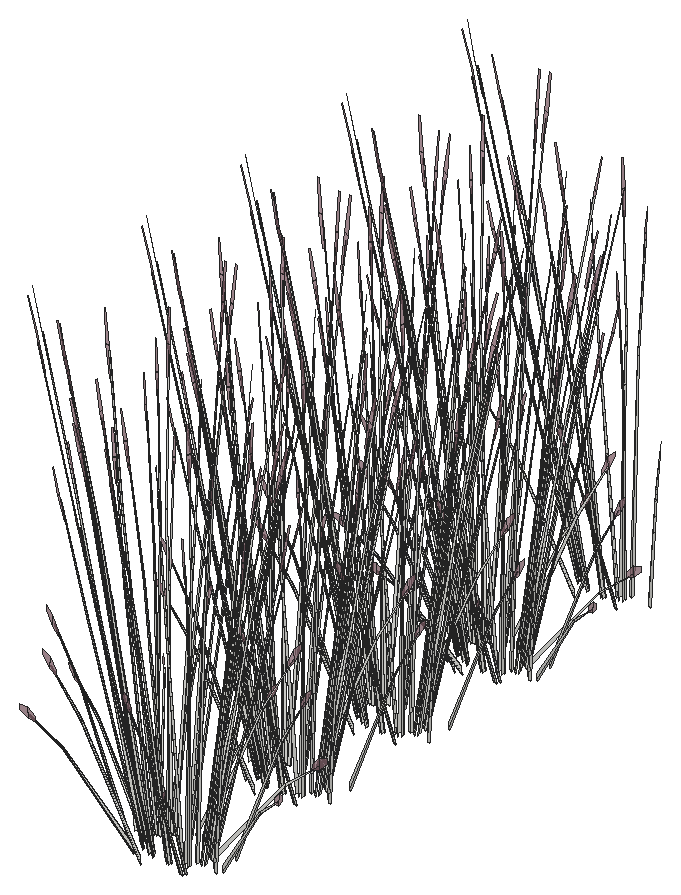
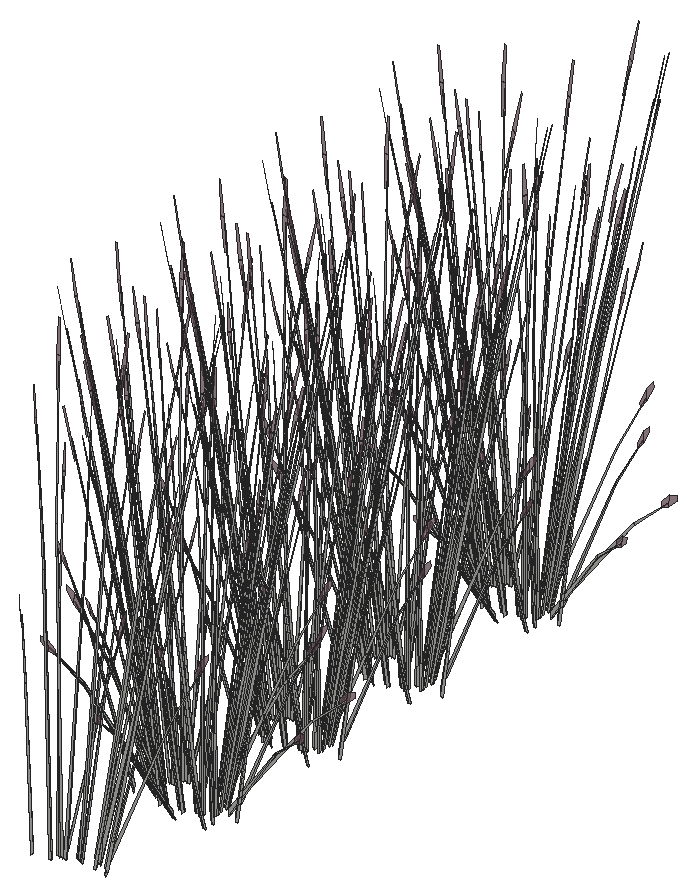
# SketchUp Ruby script. Lengths in inches.
U = 1.inch
M = Sketchup.active_model
def pt(a) = Geom::Point3d.new(a.map { |v| v * U })
def face(e, loops, mat)
  f = e.add_face(loops[0].map { |a| pt(a) })
  loops[1..].each { |l| e.add_face(l.map { |a| pt(a) }).erase! }
  f.material = f.back_material = mat if mat
  f
end
# faces: each face lists its corners as indices into pts; further lists are holes
def faces(e, pts, list, mat = nil) = list.each { |f| face(e, (f[0].is_a?(Array) ? f : [f]).map { |l| l.map { |i| pts[i] } }, mat) }
# xy, xz, yz: faces in a plane at the given z, y or x. An outline is a flat list of corners, or four numbers for a rectangle; further outlines are holes
def ring(l) = l.size == 4 ? [[l[0], l[1]], [l[2], l[1]], [l[2], l[3]], [l[0], l[3]]] : l.each_slice(2).to_a
def flat(e, list, mat, &to3) = list.each { |f| face(e, (f[0].is_a?(Array) ? f : [f]).map { |l| ring(l).map { |u, v| to3.(u, v) } }, mat) }
def xy(e, z, list, mat = nil) = flat(e, list, mat) { |x, y| [x, y, z] }
def xz(e, y, list, mat = nil) = flat(e, list, mat) { |x, z| [x, y, z] }
def yz(e, x, list, mat = nil) = flat(e, list, mat) { |y, z| [x, y, z] }
def lines(e, pts, list) = list.each { |a, b| e.add_line(pt(pts[a]), pt(pts[b])) }
# prism: a flat outline (further loops are holes) pulled along v
def prism(e, loops, v, mat = nil)
  f = face(e, loops, mat); d = Geom::Vector3d.new(v.map { |x| x * U })
  f.pushpull(f.normal.samedirection?(d) ? d.length : -d.length)
end
def box(e, o, s, mat = nil) = prism(e, [[o, [o[0] + s[0], o[1], o[2]], [o[0] + s[0], o[1] + s[1], o[2]], [o[0], o[1] + s[1], o[2]]]], [0, 0, s[2]], mat)
def at(x, y, z, deg = 0) = Geom::Transformation.translation(pt([x, y, z])) * Geom::Transformation.rotation(ORIGIN, Z_AXIS, deg.degrees)
def axes(o, x, y, z) = Geom::Transformation.new([*x, 0, *y, 0, *z, 0, *pt(o).to_a, 1])
def part(name) = M.definitions.add(name)
# library, detail: a bought-in or finely detailed component or shape, given as its bounding box
def library(name, o, s) = part(name).tap { |d| box(d.entities, o, s) }
def detail(e, o, s) = box(e.add_group.entities, o, s)
def put(e, d, t, mat = nil) = e.add_instance(d, t).tap { |i| i.material = mat if mat }
def group(e, t, mat = nil) = e.add_group.tap { |g| g.transformation = t; g.material = mat if mat }.entities
root = M.entities
M.materials.add("LightPink_Translucent").color = [144, 107, 117]
M.materials["LightPink_Translucent"].alpha = 0.75
c1 = part("blade")
p = [[2.15,0.21,22],[0,0.17,0],[0.09,0.45,0],[2.18,0.31,22],[2.29,0.31,22],[0.38,0.45,0],
  [2.48,0.24,33],[2.49,0.24,33],[2.48,0.22,33]]
faces(c1.entities,p,[[0,1,2,3],[4,5,2,3],[6,3,4,7],[8,0,3,6]])
c2 = part("seeds")
p = [[0.3,-0.1,1.38],[-0.01,-0.03,1.59],[-0.01,-0.03,0.03],[0.14,-0.07,-0.07],[0.29,-0.03,3],[0.15,0.01,3.11]]
faces(c2.entities,p,[[0,1,2,3],[1,0,4,5]],"LightPink_Translucent")
c3 = part("blade with seeds")
put(c3.entities,c1,at(0,0,0))
put(c3.entities,c2,axes([2.4,0.25,30.99],[1.5799,-0.05474,1.17369],[-0.12525,1.92788,0.29478],[-0.07173,-0.02425,1.56792]))
put(root,c3,axes([335.89,344.47,52.17],[-0.00487,-0.07777,1.54581],[-0.41166,-0.22476,-0.24447],[0.06364,-0.13625,0.12397]))
put(root,c3,axes([335.78,344.1875,52.16],[-0.05128,0.02985,1.56736],[-0.5024,-0.1007,-0.1481],[-0.01819,-0.13025,0.27737]))
put(root,c3,axes([333.05,343.62,52.16],[-0.00942,0.04684,1.56736],[-0.46458,0.16998,-0.1481],[-0.13671,-0.08689,0.27737]))
put(root,c3,axes([332.94,344.45,52.5],[0.56246,-0.10044,0.47505],[0.09762,0.39398,0.3917],[-0.13228,-0.11611,0.983]))
put(root,c3,axes([334.22,344.52,52.18],[0.49753,0.10215,0.42415],[-0.17013,0.33585,0.34973],[-0.0299,-0.13207,0.87768]))
put(root,c3,axes([334.35,344.49,52.18],[0.37205,-0.1328,0.05682],[0.18211,0.24217,0.44729],[-0.03593,-0.10675,0.68204]))
put(root,c3,axes([333.07,344.53,52.18],[0.22948,-0.24822,0.05682],[0.32679,0.14452,0.44729],[-0.10565,-0.07958,0.68204]))
put(root,c3,axes([334.21,344.77,52.46],[-0.15222,0.30049,0.31292],[-0.44409,-0.08764,-0.40398],[-0.04072,-0.12098,0.77298]))
put(root,c3,axes([335.34,344.89,52.18],[0.35954,0.26661,0.42415],[-0.38183,0.22994,0.34973],[0.06632,-0.12508,0.87768]))
put(root,c3,axes([333.18,344.51,52.8],[-0.33698,0.3746,-0.12034],[-0.48801,-0.21581,-0.66795],[-0.16964,-0.10584,1.01494]))
put(root,c3,axes([335.48,344.92,52.18],[0.41493,0.01821,0.05682],[-0.01138,0.27493,0.44729],[0.04342,-0.10531,0.68204]))
put(root,c3,axes([335.17,345.11,52.46],[-0.34164,0.20573,0.31292],[-0.3234,-0.23491,-0.40398],[0.04921,-0.11936,0.77298]))
put(root,c3,axes([331.88,344.4,52.17],[-0.10864,-0.00276,1.54581],[-0.34587,0.27582,-0.24447],[-0.18454,-0.05636,0.12397]))
put(root,c3,axes([333.14,344.82,52.46],[0.07798,0.31474,0.31292],[-0.44579,0.08311,-0.40398],[-0.11974,-0.09019,0.77298]))
put(root,c3,axes([331.8,345.02,52.5],[0.41698,-0.28837,0.47505],[0.35962,0.30624,0.3917],[-0.19563,-0.05319,0.983]))
put(root,c3,axes([337.14,345.68,52.16],[-0.06595,-0.00297,1.56736],[-0.27386,-0.31799,-0.1481],[0.10998,-0.10455,0.27737]))
put(root,c3,axes([331.99,345.02,52.18],[0.02542,-0.29714,0.05682],[0.38391,0.00815,0.44729],[-0.14706,-0.03109,0.68204]))
put(root,c3,axes([335.76,345.74,52.46],[-0.43951,0.05584,0.31292],[-0.11606,-0.31924,-0.40398],[0.12595,-0.08575,0.77298]))
put(root,c3,axes([336.16,345.69,52.18],[0.34663,0.16434,0.05682],[-0.20181,0.23402,0.44729],[0.11113,-0.07566,0.68204]))
put(root,c3,axes([336.0625,345.62,52.18],[0.12522,0.35963,0.42415],[-0.49122,0.06241,0.34973],[0.14477,-0.08458,0.87768]))
put(root,c3,axes([337.39,346.06,52.17],[0.07006,-0.05952,1.54581],[-0.08968,-0.3651,-0.24447],[0.1758,-0.06922,0.12397]))
put(root,c3,axes([331.47,344.63,52.16],[0.03743,0.039,1.56736],[-0.18045,0.35054,-0.1481],[-0.18276,0.00254,0.27737]))
put(root,c3,axes([332.25,345.24,52.46],[0.28729,0.24465,0.31292],[-0.32804,0.23159,-0.40398],[-0.16667,-0.03524,0.77298]))
put(root,c3,axes([335.83,346.5,52.46],[-0.41962,-0.10901,0.31292],[0.12239,-0.31802,-0.40398],[0.16894,-0.02916,0.77298]))
put(root,c3,axes([331.4375,345.92,52.18],[0.14265,-0.35629,0.42415],[0.46898,0.12183,0.34973],[-0.18443,0.02141,0.87768]))
put(root,c3,axes([331.4,345.83,52.18],[-0.18545,-0.26643,0.05682],[0.33817,-0.13041,0.44729],[-0.14907,0.02573,0.68204]))
put(root,c3,axes([336.21,346.6,52.18],[0.18545,0.26643,0.05682],[-0.33817,0.13041,0.44729],[0.14907,-0.02573,0.68204]))
put(root,c3,axes([336.18,346.51,52.18],[-0.14265,0.35629,0.42415],[-0.46898,-0.12183,0.34973],[0.18443,-0.02141,0.87768]))
put(root,c3,axes([331.78,345.93,52.46],[0.41962,0.10901,0.31292],[-0.12239,0.31802,-0.40398],[-0.16894,0.02916,0.77298]))
put(root,c3,axes([337.02,347.66,52.16],[-0.04566,-0.03421,1.56736],[0.09987,-0.36669,-0.1481],[0.17984,-0.02343,0.27737]))
put(root,c3,axes([331.08,346.17,52.17],[-0.08245,0.05073,1.54581],[0.00701,0.37067,-0.24447],[-0.18899,0.0482,0.12397]))
put(root,c3,axes([335.36,347.19,52.46],[-0.28729,-0.24465,0.31292],[0.32804,-0.23159,-0.40398],[0.16667,0.03524,0.77298]))
put(root,c3,axes([335.88,347.11,52.17],[0.10831,-0.00661,1.54581],[0.29709,-0.30358,-0.24447],[0.19266,0.04007,0.12397]))
put(root,c3,axes([331.55,346.8125,52.18],[-0.12522,-0.35963,0.42415],[0.49122,-0.06241,0.34973],[-0.14477,0.08458,0.87768]))
put(root,c3,axes([331.45,346.74,52.18],[-0.34663,-0.16434,0.05682],[0.20181,-0.23402,0.44729],[-0.11113,0.07566,0.68204]))
put(root,c3,axes([331.85,346.69,52.46],[0.43951,-0.05584,0.31292],[0.11606,0.31924,-0.40398],[-0.12595,0.08575,0.77298]))
put(root,c3,axes([330.16,346.55,52.16],[0.06444,0.01048,1.56736],[0.19934,0.34525,-0.1481],[-0.13191,0.09062,0.27737]))
put(root,c3,axes([335.62,347.41,52.18],[-0.02542,0.29714,0.05682],[-0.38391,-0.00815,0.44729],[0.14706,0.03109,0.68204]))
put(root,c3,axes([335.65,347.32,52.18],[-0.3723,0.25748,0.42415],[-0.32109,-0.27343,0.34973],[0.17467,0.04749,0.87768]))
put(root,c3,axes([330.85,347.6,52.99],[0.44556,0.1043,-0.05733],[-0.13706,0.32103,-0.25992],[-0.07288,0.04874,0.85731]))
put(root,c3,axes([334.47,347.62,52.46],[-0.07798,-0.31474,0.31292],[0.44579,-0.08311,-0.40398],[0.11974,0.09019,0.77298]))
put(root,c3,axes([332.45,347.33,52.46],[0.34164,-0.20573,0.31292],[0.3234,0.23491,-0.40398],[-0.04921,0.11936,0.77298]))
put(root,c3,axes([334.04,348.06,52.16],[0.00149,-0.04731,1.56736],[0.4327,-0.20872,-0.1481],[0.1503,0.0745,0.27737]))
put(root,c3,axes([332.14,347.51,52.18],[-0.41493,-0.01821,0.05682],[0.01138,-0.27493,0.44729],[-0.04342,0.10531,0.68204]))
put(root,c3,axes([332.27,347.54,52.18],[-0.35954,-0.26661,0.42415],[0.38183,-0.22994,0.34973],[-0.06632,0.12508,0.87768]))
put(root,c3,axes([333.4,347.67,52.46],[0.15222,-0.30049,0.31292],[0.44409,0.08764,-0.40398],[0.04072,0.12098,0.77298]))
put(root,c3,axes([334.54,347.9,52.18],[-0.22948,0.24822,0.05682],[-0.32679,-0.14452,0.44729],[0.10565,0.07958,0.68204]))
put(root,c3,axes([334,348.74,52.99],[0.34892,-0.22417,-0.05733],[0.3197,0.24551,-0.25992],[0.02251,0.06957,0.85731]))
put(root,c3,axes([334.64,347.83,52.18],[-0.5022,0.08967,0.42415],[-0.08716,-0.35177,0.34973],[0.11811,0.10367,0.87768]))
put(root,c3,axes([333.27,347.9375,52.18],[-0.37205,0.1328,0.05682],[-0.18211,-0.24217,0.44729],[0.03593,0.10675,0.68204]))
put(root,c3,axes([331.09,347.56,52.17],[-0.01255,0.07733,1.54581],[0.35618,0.269,-0.24447],[-0.09325,0.12721,0.12397]))
put(root,c3,axes([332.23,347.38,52.77],[0.55492,0.01936,-0.11927],[-0.01517,0.36657,-0.66198],[-0.03855,0.14118,1.00587]))
put(root,c3,axes([333.4,347.91,52.47],[-0.49753,-0.10215,0.47081],[0.17013,-0.33585,0.3882],[0.0299,0.13207,0.97422]))
put(root,c3,axes([331.05,348.35,52.16],[0.05728,-0.02359,1.56736],[0.47345,0.15692,-0.1481],[-0.01113,0.13066,0.27737]))
put(root,c3,axes([333.14,348.51,52.17],[0.064,0.06292,1.54581],[0.51651,0.02472,-0.24447],[0.05194,0.13877,0.12397]))
put(root,c3,axes([335.78,354.91,52.16],[-0.05128,0.02985,1.56736],[-0.5024,-0.1007,-0.1481],[-0.01819,-0.13025,0.27737]))
put(root,c3,axes([333.05,354.34,52.16],[-0.00942,0.04684,1.56736],[-0.46458,0.16998,-0.1481],[-0.13671,-0.08689,0.27737]))
put(root,c3,axes([332.94,355.17,52.5],[0.56246,-0.10044,0.47505],[0.09762,0.39398,0.3917],[-0.13228,-0.11611,0.983]))
put(root,c3,axes([334.22,355.24,52.18],[0.49753,0.10215,0.42415],[-0.17013,0.33585,0.34973],[-0.0299,-0.13207,0.87768]))
put(root,c3,axes([334.35,355.22,52.18],[0.37205,-0.1328,0.05682],[0.18211,0.24217,0.44729],[-0.03593,-0.10675,0.68204]))
put(root,c3,axes([333.07,355.25,52.18],[0.22948,-0.24822,0.05682],[0.32679,0.14452,0.44729],[-0.10565,-0.07958,0.68204]))
put(root,c3,axes([334.21,355.49,52.46],[-0.15222,0.30049,0.31292],[-0.44409,-0.08764,-0.40398],[-0.04072,-0.12098,0.77298]))
put(root,c3,axes([335.34,355.62,52.18],[0.35954,0.26661,0.42415],[-0.38183,0.22994,0.34973],[0.06632,-0.12508,0.87768]))
put(root,c3,axes([333.18,355.23,52.8],[-0.33698,0.3746,-0.12034],[-0.48801,-0.21581,-0.66795],[-0.16964,-0.10584,1.01494]))
put(root,c3,axes([335.48,355.64,52.18],[0.41493,0.01821,0.05682],[-0.01138,0.27493,0.44729],[0.04342,-0.10531,0.68204]))
put(root,c3,axes([335.17,355.83,52.46],[-0.34164,0.20573,0.31292],[-0.3234,-0.23491,-0.40398],[0.04921,-0.11936,0.77298]))
put(root,c3,axes([333.14,355.54,52.46],[0.07798,0.31474,0.31292],[-0.44579,0.08311,-0.40398],[-0.11974,-0.09019,0.77298]))
put(root,c3,axes([331.8,355.74,52.5],[0.41698,-0.28837,0.47505],[0.35962,0.30624,0.3917],[-0.19563,-0.05319,0.983]))
put(root,c3,axes([337.14,356.4,52.16],[-0.06595,-0.00297,1.56736],[-0.27386,-0.31799,-0.1481],[0.10998,-0.10455,0.27737]))
put(root,c3,axes([331.99,355.74,52.18],[0.02542,-0.29714,0.05682],[0.38391,0.00815,0.44729],[-0.14706,-0.03109,0.68204]))
put(root,c3,axes([335.76,356.46,52.46],[-0.43951,0.05584,0.31292],[-0.11606,-0.31924,-0.40398],[0.12595,-0.08575,0.77298]))
put(root,c3,axes([336.16,356.41,52.18],[0.34663,0.16434,0.05682],[-0.20181,0.23402,0.44729],[0.11113,-0.07566,0.68204]))
put(root,c3,axes([336.0625,356.34,52.18],[0.12522,0.35963,0.42415],[-0.49122,0.06241,0.34973],[0.14477,-0.08458,0.87768]))
put(root,c3,axes([331.47,355.35,52.16],[0.03743,0.039,1.56736],[-0.18045,0.35054,-0.1481],[-0.18276,0.00254,0.27737]))
put(root,c3,axes([332.25,355.96,52.46],[0.28729,0.24465,0.31292],[-0.32804,0.23159,-0.40398],[-0.16667,-0.03524,0.77298]))
put(root,c3,axes([335.83,357.23,52.46],[-0.41962,-0.10901,0.31292],[0.12239,-0.31802,-0.40398],[0.16894,-0.02916,0.77298]))
put(root,c3,axes([331.4375,356.65,52.18],[0.14265,-0.35629,0.42415],[0.46898,0.12183,0.34973],[-0.18443,0.02141,0.87768]))
put(root,c3,axes([331.4,356.55,52.18],[-0.18545,-0.26643,0.05682],[0.33817,-0.13041,0.44729],[-0.14907,0.02573,0.68204]))
put(root,c3,axes([336.21,357.33,52.18],[0.18545,0.26643,0.05682],[-0.33817,0.13041,0.44729],[0.14907,-0.02573,0.68204]))
put(root,c3,axes([336.18,357.23,52.18],[-0.14265,0.35629,0.42415],[-0.46898,-0.12183,0.34973],[0.18443,-0.02141,0.87768]))
put(root,c3,axes([331.78,356.65,52.46],[0.41962,0.10901,0.31292],[-0.12239,0.31802,-0.40398],[-0.16894,0.02916,0.77298]))
put(root,c3,axes([337.02,358.38,52.16],[-0.04566,-0.03421,1.56736],[0.09987,-0.36669,-0.1481],[0.17984,-0.02343,0.27737]))
put(root,c3,axes([335.36,357.91,52.46],[-0.28729,-0.24465,0.31292],[0.32804,-0.23159,-0.40398],[0.16667,0.03524,0.77298]))
put(root,c3,axes([331.55,357.53,52.18],[-0.12522,-0.35963,0.42415],[0.49122,-0.06241,0.34973],[-0.14477,0.08458,0.87768]))
put(root,c3,axes([331.45,357.46,52.18],[-0.34663,-0.16434,0.05682],[0.20181,-0.23402,0.44729],[-0.11113,0.07566,0.68204]))
put(root,c3,axes([331.85,357.41,52.46],[0.43951,-0.05584,0.31292],[0.11606,0.31924,-0.40398],[-0.12595,0.08575,0.77298]))
put(root,c3,axes([330.16,357.27,52.16],[0.06444,0.01048,1.56736],[0.19934,0.34525,-0.1481],[-0.13191,0.09062,0.27737]))
put(root,c3,axes([335.62,358.13,52.18],[-0.02542,0.29714,0.05682],[-0.38391,-0.00815,0.44729],[0.14706,0.03109,0.68204]))
put(root,c3,axes([335.65,358.04,52.18],[-0.3723,0.25748,0.42415],[-0.32109,-0.27343,0.34973],[0.17467,0.04749,0.87768]))
put(root,c3,axes([330.85,358.32,52.99],[0.44556,0.1043,-0.05733],[-0.13706,0.32103,-0.25992],[-0.07288,0.04874,0.85731]))
put(root,c3,axes([334.47,358.34,52.46],[-0.07798,-0.31474,0.31292],[0.44579,-0.08311,-0.40398],[0.11974,0.09019,0.77298]))
put(root,c3,axes([332.45,358.05,52.46],[0.34164,-0.20573,0.31292],[0.3234,0.23491,-0.40398],[-0.04921,0.11936,0.77298]))
put(root,c3,axes([334.04,358.78,52.16],[0.00149,-0.04731,1.56736],[0.4327,-0.20872,-0.1481],[0.1503,0.0745,0.27737]))
put(root,c3,axes([332.14,358.24,52.18],[-0.41493,-0.01821,0.05682],[0.01138,-0.27493,0.44729],[-0.04342,0.10531,0.68204]))
put(root,c3,axes([332.27,358.26,52.18],[-0.35954,-0.26661,0.42415],[0.38183,-0.22994,0.34973],[-0.06632,0.12508,0.87768]))
put(root,c3,axes([333.4,358.39,52.46],[0.15222,-0.30049,0.31292],[0.44409,0.08764,-0.40398],[0.04072,0.12098,0.77298]))
put(root,c3,axes([334.54,358.625,52.18],[-0.22948,0.24822,0.05682],[-0.32679,-0.14452,0.44729],[0.10565,0.07958,0.68204]))
put(root,c3,axes([334,359.46,52.99],[0.34892,-0.22417,-0.05733],[0.3197,0.24551,-0.25992],[0.02251,0.06957,0.85731]))
put(root,c3,axes([334.64,358.55,52.18],[-0.5022,0.08967,0.42415],[-0.08716,-0.35177,0.34973],[0.11811,0.10367,0.87768]))
put(root,c3,axes([333.27,358.66,52.18],[-0.37205,0.1328,0.05682],[-0.18211,-0.24217,0.44729],[0.03593,0.10675,0.68204]))
put(root,c3,axes([332.23,358.11,52.77],[0.55492,0.01936,-0.11927],[-0.01517,0.36657,-0.66198],[-0.03855,0.14118,1.00587]))
put(root,c3,axes([333.4,358.63,52.47],[-0.49753,-0.10215,0.47081],[0.17013,-0.33585,0.3882],[0.0299,0.13207,0.97422]))
put(root,c3,axes([331.05,359.07,52.16],[0.05728,-0.02359,1.56736],[0.47345,0.15692,-0.1481],[-0.01113,0.13066,0.27737]))
put(root,c3,axes([335.78,364.24,52.16],[-0.05128,0.02985,1.56736],[-0.5024,-0.1007,-0.1481],[-0.01819,-0.13025,0.27737]))
put(root,c3,axes([333.05,363.66,52.16],[-0.00942,0.04684,1.56736],[-0.46458,0.16998,-0.1481],[-0.13671,-0.08689,0.27737]))
put(root,c3,axes([332.94,364.49,52.5],[0.56246,-0.10044,0.47505],[0.09762,0.39398,0.3917],[-0.13228,-0.11611,0.983]))
put(root,c3,axes([334.22,364.57,52.18],[0.49753,0.10215,0.42415],[-0.17013,0.33585,0.34973],[-0.0299,-0.13207,0.87768]))
put(root,c3,axes([334.35,364.54,52.18],[0.37205,-0.1328,0.05682],[0.18211,0.24217,0.44729],[-0.03593,-0.10675,0.68204]))
put(root,c3,axes([333.07,364.58,52.18],[0.22948,-0.24822,0.05682],[0.32679,0.14452,0.44729],[-0.10565,-0.07958,0.68204]))
put(root,c3,axes([334.21,364.82,52.46],[-0.15222,0.30049,0.31292],[-0.44409,-0.08764,-0.40398],[-0.04072,-0.12098,0.77298]))
put(root,c3,axes([335.34,364.94,52.18],[0.35954,0.26661,0.42415],[-0.38183,0.22994,0.34973],[0.06632,-0.12508,0.87768]))
put(root,c3,axes([333.18,364.55,52.8],[-0.33698,0.3746,-0.12034],[-0.48801,-0.21581,-0.66795],[-0.16964,-0.10584,1.01494]))
put(root,c3,axes([335.48,364.97,52.18],[0.41493,0.01821,0.05682],[-0.01138,0.27493,0.44729],[0.04342,-0.10531,0.68204]))
put(root,c3,axes([335.17,365.15,52.46],[-0.34164,0.20573,0.31292],[-0.3234,-0.23491,-0.40398],[0.04921,-0.11936,0.77298]))
put(root,c3,axes([333.14,364.87,52.46],[0.07798,0.31474,0.31292],[-0.44579,0.08311,-0.40398],[-0.11974,-0.09019,0.77298]))
put(root,c3,axes([331.8,365.07,52.5],[0.41698,-0.28837,0.47505],[0.35962,0.30624,0.3917],[-0.19563,-0.05319,0.983]))
put(root,c3,axes([337.14,365.73,52.16],[-0.06595,-0.00297,1.56736],[-0.27386,-0.31799,-0.1481],[0.10998,-0.10455,0.27737]))
put(root,c3,axes([331.99,365.07,52.18],[0.02542,-0.29714,0.05682],[0.38391,0.00815,0.44729],[-0.14706,-0.03109,0.68204]))
put(root,c3,axes([335.76,365.79,52.46],[-0.43951,0.05584,0.31292],[-0.11606,-0.31924,-0.40398],[0.12595,-0.08575,0.77298]))
put(root,c3,axes([336.16,365.74,52.18],[0.34663,0.16434,0.05682],[-0.20181,0.23402,0.44729],[0.11113,-0.07566,0.68204]))
put(root,c3,axes([336.0625,365.67,52.18],[0.12522,0.35963,0.42415],[-0.49122,0.06241,0.34973],[0.14477,-0.08458,0.87768]))
put(root,c3,axes([331.47,364.68,52.16],[0.03743,0.039,1.56736],[-0.18045,0.35054,-0.1481],[-0.18276,0.00254,0.27737]))
put(root,c3,axes([332.25,365.29,52.46],[0.28729,0.24465,0.31292],[-0.32804,0.23159,-0.40398],[-0.16667,-0.03524,0.77298]))
put(root,c3,axes([335.83,366.55,52.46],[-0.41962,-0.10901,0.31292],[0.12239,-0.31802,-0.40398],[0.16894,-0.02916,0.77298]))
put(root,c3,axes([331.4375,365.97,52.18],[0.14265,-0.35629,0.42415],[0.46898,0.12183,0.34973],[-0.18443,0.02141,0.87768]))
put(root,c3,axes([331.4,365.88,52.18],[-0.18545,-0.26643,0.05682],[0.33817,-0.13041,0.44729],[-0.14907,0.02573,0.68204]))
put(root,c3,axes([336.21,366.65,52.18],[0.18545,0.26643,0.05682],[-0.33817,0.13041,0.44729],[0.14907,-0.02573,0.68204]))
put(root,c3,axes([336.18,366.56,52.18],[-0.14265,0.35629,0.42415],[-0.46898,-0.12183,0.34973],[0.18443,-0.02141,0.87768]))
put(root,c3,axes([331.78,365.98,52.46],[0.41962,0.10901,0.31292],[-0.12239,0.31802,-0.40398],[-0.16894,0.02916,0.77298]))
put(root,c3,axes([337.02,367.71,52.16],[-0.04566,-0.03421,1.56736],[0.09987,-0.36669,-0.1481],[0.17984,-0.02343,0.27737]))
put(root,c3,axes([335.36,367.24,52.46],[-0.28729,-0.24465,0.31292],[0.32804,-0.23159,-0.40398],[0.16667,0.03524,0.77298]))
put(root,c3,axes([331.55,366.86,52.18],[-0.12522,-0.35963,0.42415],[0.49122,-0.06241,0.34973],[-0.14477,0.08458,0.87768]))
put(root,c3,axes([331.45,366.79,52.18],[-0.34663,-0.16434,0.05682],[0.20181,-0.23402,0.44729],[-0.11113,0.07566,0.68204]))
put(root,c3,axes([331.85,366.74,52.46],[0.43951,-0.05584,0.31292],[0.11606,0.31924,-0.40398],[-0.12595,0.08575,0.77298]))
put(root,c3,axes([330.16,366.6,52.16],[0.06444,0.01048,1.56736],[0.19934,0.34525,-0.1481],[-0.13191,0.09062,0.27737]))
put(root,c3,axes([335.62,367.46,52.18],[-0.02542,0.29714,0.05682],[-0.38391,-0.00815,0.44729],[0.14706,0.03109,0.68204]))
put(root,c3,axes([335.65,367.37,52.18],[-0.3723,0.25748,0.42415],[-0.32109,-0.27343,0.34973],[0.17467,0.04749,0.87768]))
put(root,c3,axes([330.85,367.65,52.99],[0.44556,0.1043,-0.05733],[-0.13706,0.32103,-0.25992],[-0.07288,0.04874,0.85731]))
put(root,c3,axes([334.47,367.66,52.46],[-0.07798,-0.31474,0.31292],[0.44579,-0.08311,-0.40398],[0.11974,0.09019,0.77298]))
put(root,c3,axes([332.45,367.375,52.46],[0.34164,-0.20573,0.31292],[0.3234,0.23491,-0.40398],[-0.04921,0.11936,0.77298]))
put(root,c3,axes([334.04,368.1,52.16],[0.00149,-0.04731,1.56736],[0.4327,-0.20872,-0.1481],[0.1503,0.0745,0.27737]))
put(root,c3,axes([332.14,367.5625,52.18],[-0.41493,-0.01821,0.05682],[0.01138,-0.27493,0.44729],[-0.04342,0.10531,0.68204]))
put(root,c3,axes([332.27,367.59,52.18],[-0.35954,-0.26661,0.42415],[0.38183,-0.22994,0.34973],[-0.06632,0.12508,0.87768]))
put(root,c3,axes([333.4,367.71,52.46],[0.15222,-0.30049,0.31292],[0.44409,0.08764,-0.40398],[0.04072,0.12098,0.77298]))
put(root,c3,axes([334.54,367.95,52.18],[-0.22948,0.24822,0.05682],[-0.32679,-0.14452,0.44729],[0.10565,0.07958,0.68204]))
put(root,c3,axes([334,368.79,52.99],[0.34892,-0.22417,-0.05733],[0.3197,0.24551,-0.25992],[0.02251,0.06957,0.85731]))
put(root,c3,axes([334.64,367.88,52.18],[-0.5022,0.08967,0.42415],[-0.08716,-0.35177,0.34973],[0.11811,0.10367,0.87768]))
put(root,c3,axes([333.27,367.99,52.18],[-0.37205,0.1328,0.05682],[-0.18211,-0.24217,0.44729],[0.03593,0.10675,0.68204]))
put(root,c3,axes([332.23,367.43,52.77],[0.55492,0.01936,-0.11927],[-0.01517,0.36657,-0.66198],[-0.03855,0.14118,1.00587]))
put(root,c3,axes([333.4,367.96,52.47],[-0.49753,-0.10215,0.47081],[0.17013,-0.33585,0.3882],[0.0299,0.13207,0.97422]))
put(root,c3,axes([331.05,368.4,52.16],[0.05728,-0.02359,1.56736],[0.47345,0.15692,-0.1481],[-0.01113,0.13066,0.27737]))
put(root,c3,axes([333.57,373.32,52.17],[-0.07723,-0.05479,1.54581],[-0.51538,0.03473,-0.24447],[-0.08225,-0.13104,0.12397]))
put(root,c3,axes([335.89,373.99,52.17],[-0.00487,-0.07777,1.54581],[-0.41166,-0.22476,-0.24447],[0.06364,-0.13625,0.12397]))
put(root,c3,axes([335.78,373.71,52.16],[-0.05128,0.02985,1.56736],[-0.5024,-0.1007,-0.1481],[-0.01819,-0.13025,0.27737]))
put(root,c3,axes([333.05,373.14,52.16],[-0.00942,0.04684,1.56736],[-0.46458,0.16998,-0.1481],[-0.13671,-0.08689,0.27737]))
put(root,c3,axes([332.94,373.97,52.5],[0.56246,-0.10044,0.47505],[0.09762,0.39398,0.3917],[-0.13228,-0.11611,0.983]))
put(root,c3,axes([334.22,374.04,52.18],[0.49753,0.10215,0.42415],[-0.17013,0.33585,0.34973],[-0.0299,-0.13207,0.87768]))
put(root,c3,axes([334.35,374.02,52.18],[0.37205,-0.1328,0.05682],[0.18211,0.24217,0.44729],[-0.03593,-0.10675,0.68204]))
put(root,c3,axes([333.07,374.05,52.18],[0.22948,-0.24822,0.05682],[0.32679,0.14452,0.44729],[-0.10565,-0.07958,0.68204]))
put(root,c3,axes([334.21,374.29,52.46],[-0.15222,0.30049,0.31292],[-0.44409,-0.08764,-0.40398],[-0.04072,-0.12098,0.77298]))
put(root,c3,axes([335.34,374.41,52.18],[0.35954,0.26661,0.42415],[-0.38183,0.22994,0.34973],[0.06632,-0.12508,0.87768]))
put(root,c3,axes([333.18,374.03,52.8],[-0.33698,0.3746,-0.12034],[-0.48801,-0.21581,-0.66795],[-0.16964,-0.10584,1.01494]))
put(root,c3,axes([335.48,374.4375,52.18],[0.41493,0.01821,0.05682],[-0.01138,0.27493,0.44729],[0.04342,-0.10531,0.68204]))
put(root,c3,axes([335.17,374.625,52.46],[-0.34164,0.20573,0.31292],[-0.3234,-0.23491,-0.40398],[0.04921,-0.11936,0.77298]))
put(root,c3,axes([331.88,373.92,52.17],[-0.10864,-0.00276,1.54581],[-0.34587,0.27582,-0.24447],[-0.18454,-0.05636,0.12397]))
put(root,c3,axes([333.14,374.34,52.46],[0.07798,0.31474,0.31292],[-0.44579,0.08311,-0.40398],[-0.11974,-0.09019,0.77298]))
put(root,c3,axes([331.8,374.54,52.5],[0.41698,-0.28837,0.47505],[0.35962,0.30624,0.3917],[-0.19563,-0.05319,0.983]))
put(root,c3,axes([337.14,375.2,52.16],[-0.06595,-0.00297,1.56736],[-0.27386,-0.31799,-0.1481],[0.10998,-0.10455,0.27737]))
put(root,c3,axes([331.99,374.54,52.18],[0.02542,-0.29714,0.05682],[0.38391,0.00815,0.44729],[-0.14706,-0.03109,0.68204]))
put(root,c3,axes([335.76,375.26,52.46],[-0.43951,0.05584,0.31292],[-0.11606,-0.31924,-0.40398],[0.12595,-0.08575,0.77298]))
put(root,c3,axes([336.16,375.21,52.18],[0.34663,0.16434,0.05682],[-0.20181,0.23402,0.44729],[0.11113,-0.07566,0.68204]))
put(root,c3,axes([336.0625,375.14,52.18],[0.12522,0.35963,0.42415],[-0.49122,0.06241,0.34973],[0.14477,-0.08458,0.87768]))
put(root,c3,axes([337.39,375.58,52.17],[0.07006,-0.05952,1.54581],[-0.08968,-0.3651,-0.24447],[0.1758,-0.06922,0.12397]))
put(root,c3,axes([331.47,374.15,52.16],[0.03743,0.039,1.56736],[-0.18045,0.35054,-0.1481],[-0.18276,0.00254,0.27737]))
put(root,c3,axes([332.25,374.76,52.46],[0.28729,0.24465,0.31292],[-0.32804,0.23159,-0.40398],[-0.16667,-0.03524,0.77298]))
put(root,c3,axes([335.83,376.03,52.46],[-0.41962,-0.10901,0.31292],[0.12239,-0.31802,-0.40398],[0.16894,-0.02916,0.77298]))
put(root,c3,axes([331.4375,375.44,52.18],[0.14265,-0.35629,0.42415],[0.46898,0.12183,0.34973],[-0.18443,0.02141,0.87768]))
put(root,c3,axes([331.4,375.35,52.18],[-0.18545,-0.26643,0.05682],[0.33817,-0.13041,0.44729],[-0.14907,0.02573,0.68204]))
put(root,c3,axes([336.21,376.125,52.18],[0.18545,0.26643,0.05682],[-0.33817,0.13041,0.44729],[0.14907,-0.02573,0.68204]))
put(root,c3,axes([336.18,376.03,52.18],[-0.14265,0.35629,0.42415],[-0.46898,-0.12183,0.34973],[0.18443,-0.02141,0.87768]))
put(root,c3,axes([331.78,375.45,52.46],[0.41962,0.10901,0.31292],[-0.12239,0.31802,-0.40398],[-0.16894,0.02916,0.77298]))
put(root,c3,axes([337.02,377.18,52.16],[-0.04566,-0.03421,1.56736],[0.09987,-0.36669,-0.1481],[0.17984,-0.02343,0.27737]))
put(root,c3,axes([331.08,375.7,52.17],[-0.08245,0.05073,1.54581],[0.00701,0.37067,-0.24447],[-0.18899,0.0482,0.12397]))
put(root,c3,axes([335.36,376.71,52.46],[-0.28729,-0.24465,0.31292],[0.32804,-0.23159,-0.40398],[0.16667,0.03524,0.77298]))
put(root,c3,axes([335.88,376.63,52.17],[0.10831,-0.00661,1.54581],[0.29709,-0.30358,-0.24447],[0.19266,0.04007,0.12397]))
put(root,c3,axes([331.55,376.33,52.18],[-0.12522,-0.35963,0.42415],[0.49122,-0.06241,0.34973],[-0.14477,0.08458,0.87768]))
put(root,c3,axes([331.45,376.26,52.18],[-0.34663,-0.16434,0.05682],[0.20181,-0.23402,0.44729],[-0.11113,0.07566,0.68204]))
put(root,c3,axes([331.85,376.21,52.46],[0.43951,-0.05584,0.31292],[0.11606,0.31924,-0.40398],[-0.12595,0.08575,0.77298]))
put(root,c3,axes([330.16,376.07,52.16],[0.06444,0.01048,1.56736],[0.19934,0.34525,-0.1481],[-0.13191,0.09062,0.27737]))
put(root,c3,axes([335.62,376.93,52.18],[-0.02542,0.29714,0.05682],[-0.38391,-0.00815,0.44729],[0.14706,0.03109,0.68204]))
put(root,c3,axes([335.65,376.84,52.18],[-0.3723,0.25748,0.42415],[-0.32109,-0.27343,0.34973],[0.17467,0.04749,0.87768]))
put(root,c3,axes([330.85,377.12,52.99],[0.44556,0.1043,-0.05733],[-0.13706,0.32103,-0.25992],[-0.07288,0.04874,0.85731]))
put(root,c3,axes([334.47,377.14,52.46],[-0.07798,-0.31474,0.31292],[0.44579,-0.08311,-0.40398],[0.11974,0.09019,0.77298]))
put(root,c3,axes([332.45,376.85,52.46],[0.34164,-0.20573,0.31292],[0.3234,0.23491,-0.40398],[-0.04921,0.11936,0.77298]))
put(root,c3,axes([334.04,377.58,52.16],[0.00149,-0.04731,1.56736],[0.4327,-0.20872,-0.1481],[0.1503,0.0745,0.27737]))
put(root,c3,axes([332.14,377.03,52.18],[-0.41493,-0.01821,0.05682],[0.01138,-0.27493,0.44729],[-0.04342,0.10531,0.68204]))
put(root,c3,axes([332.27,377.06,52.18],[-0.35954,-0.26661,0.42415],[0.38183,-0.22994,0.34973],[-0.06632,0.12508,0.87768]))
put(root,c3,axes([333.4,377.1875,52.46],[0.15222,-0.30049,0.31292],[0.44409,0.08764,-0.40398],[0.04072,0.12098,0.77298]))
put(root,c3,axes([334.54,377.42,52.18],[-0.22948,0.24822,0.05682],[-0.32679,-0.14452,0.44729],[0.10565,0.07958,0.68204]))
put(root,c3,axes([334,378.26,52.99],[0.34892,-0.22417,-0.05733],[0.3197,0.24551,-0.25992],[0.02251,0.06957,0.85731]))
put(root,c3,axes([334.64,377.35,52.18],[-0.5022,0.08967,0.42415],[-0.08716,-0.35177,0.34973],[0.11811,0.10367,0.87768]))
put(root,c3,axes([333.27,377.46,52.18],[-0.37205,0.1328,0.05682],[-0.18211,-0.24217,0.44729],[0.03593,0.10675,0.68204]))
put(root,c3,axes([331.09,377.08,52.17],[-0.01255,0.07733,1.54581],[0.35618,0.269,-0.24447],[-0.09325,0.12721,0.12397]))
put(root,c3,axes([332.23,376.9,52.77],[0.55492,0.01936,-0.11927],[-0.01517,0.36657,-0.66198],[-0.03855,0.14118,1.00587]))
put(root,c3,axes([333.4,377.43,52.47],[-0.49753,-0.10215,0.47081],[0.17013,-0.33585,0.3882],[0.0299,0.13207,0.97422]))
put(root,c3,axes([331.05,377.87,52.16],[0.05728,-0.02359,1.56736],[0.47345,0.15692,-0.1481],[-0.01113,0.13066,0.27737]))
put(root,c3,axes([333.14,378.04,52.17],[0.064,0.06292,1.54581],[0.51651,0.02472,-0.24447],[0.05194,0.13877,0.12397]))
put(root,c3,axes([335.78,385.02,52.16],[-0.05128,0.02985,1.56736],[-0.5024,-0.1007,-0.1481],[-0.01819,-0.13025,0.27737]))
put(root,c3,axes([333.05,384.44,52.16],[-0.00942,0.04684,1.56736],[-0.46458,0.16998,-0.1481],[-0.13671,-0.08689,0.27737]))
put(root,c3,axes([332.94,385.28,52.5],[0.56246,-0.10044,0.47505],[0.09762,0.39398,0.3917],[-0.13228,-0.11611,0.983]))
put(root,c3,axes([334.22,385.35,52.18],[0.49753,0.10215,0.42415],[-0.17013,0.33585,0.34973],[-0.0299,-0.13207,0.87768]))
put(root,c3,axes([334.35,385.32,52.18],[0.37205,-0.1328,0.05682],[0.18211,0.24217,0.44729],[-0.03593,-0.10675,0.68204]))
put(root,c3,axes([333.07,385.36,52.18],[0.22948,-0.24822,0.05682],[0.32679,0.14452,0.44729],[-0.10565,-0.07958,0.68204]))
put(root,c3,axes([334.21,385.6,52.46],[-0.15222,0.30049,0.31292],[-0.44409,-0.08764,-0.40398],[-0.04072,-0.12098,0.77298]))
put(root,c3,axes([335.34,385.72,52.18],[0.35954,0.26661,0.42415],[-0.38183,0.22994,0.34973],[0.06632,-0.12508,0.87768]))
put(root,c3,axes([333.18,385.34,52.8],[-0.33698,0.3746,-0.12034],[-0.48801,-0.21581,-0.66795],[-0.16964,-0.10584,1.01494]))
put(root,c3,axes([335.48,385.75,52.18],[0.41493,0.01821,0.05682],[-0.01138,0.27493,0.44729],[0.04342,-0.10531,0.68204]))
put(root,c3,axes([335.17,385.93,52.46],[-0.34164,0.20573,0.31292],[-0.3234,-0.23491,-0.40398],[0.04921,-0.11936,0.77298]))
put(root,c3,axes([333.14,385.65,52.46],[0.07798,0.31474,0.31292],[-0.44579,0.08311,-0.40398],[-0.11974,-0.09019,0.77298]))
put(root,c3,axes([331.8,385.85,52.5],[0.41698,-0.28837,0.47505],[0.35962,0.30624,0.3917],[-0.19563,-0.05319,0.983]))
put(root,c3,axes([337.14,386.51,52.16],[-0.06595,-0.00297,1.56736],[-0.27386,-0.31799,-0.1481],[0.10998,-0.10455,0.27737]))
put(root,c3,axes([331.99,385.85,52.18],[0.02542,-0.29714,0.05682],[0.38391,0.00815,0.44729],[-0.14706,-0.03109,0.68204]))
put(root,c3,axes([335.76,386.57,52.46],[-0.43951,0.05584,0.31292],[-0.11606,-0.31924,-0.40398],[0.12595,-0.08575,0.77298]))
